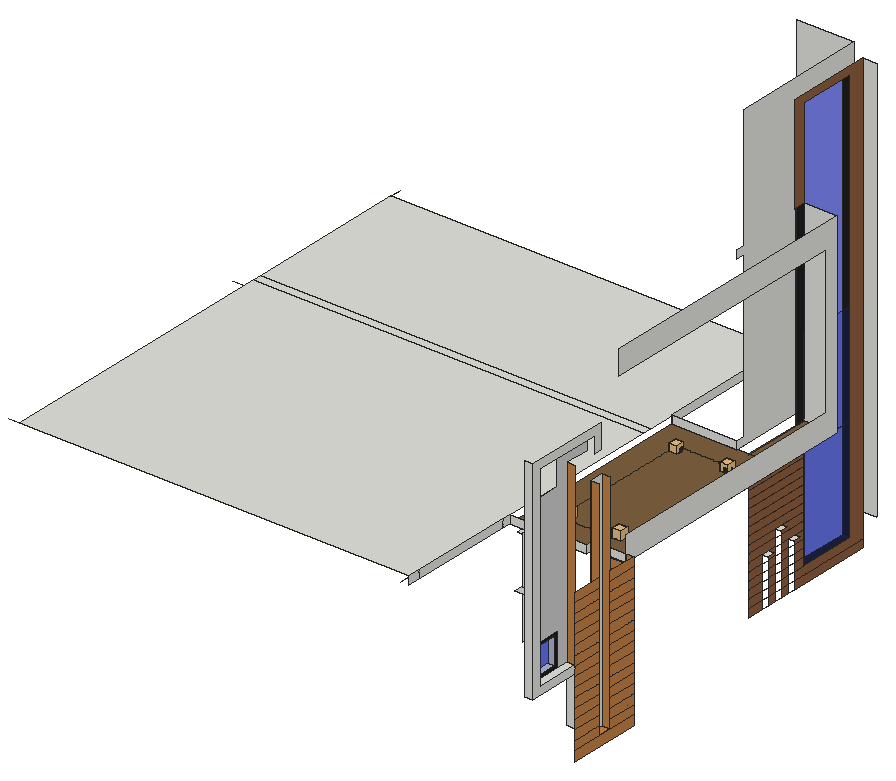
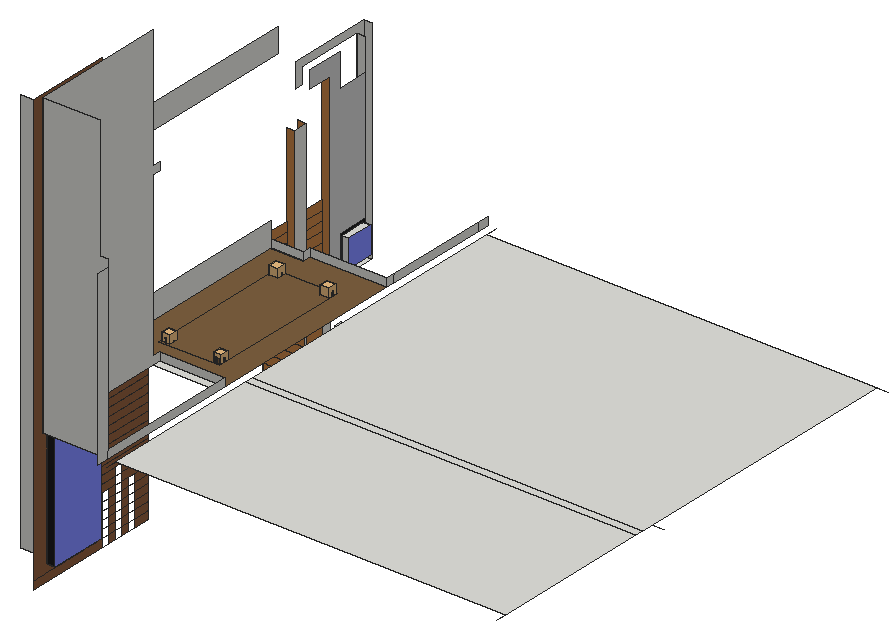
# SketchUp Ruby script. Lengths in inches.
U = 1.inch
M = Sketchup.active_model
def pt(a) = Geom::Point3d.new(a.map { |v| v * U })
def face(e, loops, mat)
  f = e.add_face(loops[0].map { |a| pt(a) })
  loops[1..].each { |l| e.add_face(l.map { |a| pt(a) }).erase! }
  f.material = f.back_material = mat if mat
  f
end
# faces: each face lists its corners as indices into pts; further lists are holes
def faces(e, pts, list, mat = nil) = list.each { |f| face(e, (f[0].is_a?(Array) ? f : [f]).map { |l| l.map { |i| pts[i] } }, mat) }
# xy, xz, yz: faces in a plane at the given z, y or x. An outline is a flat list of corners, or four numbers for a rectangle; further outlines are holes
def ring(l) = l.size == 4 ? [[l[0], l[1]], [l[2], l[1]], [l[2], l[3]], [l[0], l[3]]] : l.each_slice(2).to_a
def flat(e, list, mat, &to3) = list.each { |f| face(e, (f[0].is_a?(Array) ? f : [f]).map { |l| ring(l).map { |u, v| to3.(u, v) } }, mat) }
def xy(e, z, list, mat = nil) = flat(e, list, mat) { |x, y| [x, y, z] }
def xz(e, y, list, mat = nil) = flat(e, list, mat) { |x, z| [x, y, z] }
def yz(e, x, list, mat = nil) = flat(e, list, mat) { |y, z| [x, y, z] }
def lines(e, pts, list) = list.each { |a, b| e.add_line(pt(pts[a]), pt(pts[b])) }
# prism: a flat outline (further loops are holes) pulled along v
def prism(e, loops, v, mat = nil)
  f = face(e, loops, mat); d = Geom::Vector3d.new(v.map { |x| x * U })
  f.pushpull(f.normal.samedirection?(d) ? d.length : -d.length)
end
def box(e, o, s, mat = nil) = prism(e, [[o, [o[0] + s[0], o[1], o[2]], [o[0] + s[0], o[1] + s[1], o[2]], [o[0], o[1] + s[1], o[2]]]], [0, 0, s[2]], mat)
def at(x, y, z, deg = 0) = Geom::Transformation.translation(pt([x, y, z])) * Geom::Transformation.rotation(ORIGIN, Z_AXIS, deg.degrees)
def axes(o, x, y, z) = Geom::Transformation.new([*x, 0, *y, 0, *z, 0, *pt(o).to_a, 1])
def part(name) = M.definitions.add(name)
# library, detail: a bought-in or finely detailed component or shape, given as its bounding box
def library(name, o, s) = part(name).tap { |d| box(d.entities, o, s) }
def detail(e, o, s) = box(e.add_group.entities, o, s)
def put(e, d, t, mat = nil) = e.add_instance(d, t).tap { |i| i.material = mat if mat }
def group(e, t, mat = nil) = e.add_group.tap { |g| g.transformation = t; g.material = mat if mat }.entities
root = M.entities
M.materials.add("E01_Mint_Frost").color = [255, 255, 204]
M.materials.add("Glass_Basic_01").color = [23, 48, 186]
M.materials["Glass_Basic_01"].alpha = 0.25
M.materials.add("I03_Bluebell_Mist").color = [130, 140, 255]
M.materials.add("M08_Obsidian_Black").color = [30, 30, 30]
M.materials.add("Plywood_01_1K").color = [125, 96, 64]
M.materials.add("Wood_Floor_01_1K").color = [196, 130, 70]
M.materials.add("Wood_Veneer_15_1K").color = [142, 95, 62]
M.materials.add("[Cladding_Siding_White]1").color = [207, 207, 207]
c1 = library("Sphere Light\#7",[-3.23,-3.23,-3.23],[6.46,6.46,6.46])
c2 = library("Sphere Light\#4",[-3.22,-3.22,-3.22],[6.44,6.44,6.44])
c3 = library("Sphere Light\#6",[-2.83,-2.83,-2.83],[5.66,5.66,5.66])
c4 = library("Sphere Light\#5",[-2.98,-2.98,-2.98],[5.96,5.96,5.96])
xy(root,171.6,[[384,66.6,390,77.4]],"Wood_Floor_01_1K")
xy(root,174,[[354,294,360,336]],"M08_Obsidian_Black")
xy(root,198,[[360,255,364,261],[360,279,364,285]])
xy(root,210,[[360,267,364,273]])
xy(root,222,[[384,6,390,45]])
xy(root,228,[[384,12,390,45]])
xy(root,230,[[378.546,14,384,34]])
xy(root,231,[[312,87,342,93]],"[Cladding_Siding_White]1")
xy(root,250,[[378.546,14,384,34]])
xy(root,255.544,[[297,108,303,147],[297,151,303,188],[297,192,303,225]])
xy(root,270,[[9,9,297,225],[9,225,297,231],[9,231,297,351],[303,243,351,249]])
xy(root,270,[[[303,93,303,243,384,243,384,99,360,99,360,93],[321,117,366,225]],[[321,117,366,225],[324.799,117.348,325.568,117.497,326.272,117.84,326.864,118.353,327.302,119.002,327.557,119.743,327.613,120.524,327.464,121.293,327.121,121.997,326.607,122.588,325.958,123.027,325.218,123.282,324.437,123.337,323.668,123.188,322.964,122.845,322.372,122.332,321.934,121.683,321.679,120.943,321.624,120.161,321.773,119.393,322.115,118.688,322.629,118.097,323.278,117.659,324.018,117.403],[324.799,217.327,325.568,217.476,326.272,217.819,326.864,218.332,327.302,218.981,327.557,219.722,327.613,220.503,327.464,221.272,327.121,221.976,326.607,222.567,325.958,223.006,325.218,223.261,324.437,223.316,323.668,223.167,322.964,222.824,322.372,222.311,321.934,221.662,321.679,220.922,321.624,220.141,321.773,219.372,322.115,218.668,322.629,218.076,323.278,217.638,324.018,217.382],[362.338,217.327,363.107,217.476,363.811,217.819,364.403,218.332,364.841,218.981,365.097,219.722,365.152,220.503,365.003,221.272,364.66,221.976,364.146,222.567,363.497,223.006,362.757,223.261,361.976,223.316,361.207,223.167,360.503,222.824,359.912,222.311,359.473,221.662,359.218,220.922,359.163,220.141,359.312,219.372,359.654,218.668,360.168,218.076,360.817,217.638,361.557,217.382],[362.338,117.348,363.107,117.497,363.811,117.84,364.403,118.353,364.841,119.002,365.097,119.743,365.152,120.524,365.003,121.293,364.66,121.997,364.146,122.588,363.497,123.027,362.757,123.282,361.976,123.337,361.207,123.188,360.503,122.845,359.912,122.332,359.473,121.683,359.218,120.943,359.163,120.161,359.312,119.393,359.654,118.688,360.168,118.097,360.817,117.659,361.557,117.403]],[360,243,384,294]],"Plywood_01_1K")
xy(root,272.816,[[324.799,217.327,324.018,217.382,323.278,217.638,322.629,218.076,322.115,218.668,321.773,219.372,321.624,220.141,321.679,220.922,321.934,221.662,322.372,222.311,322.964,222.824,323.668,223.167,324.437,223.316,325.218,223.261,325.958,223.006,326.607,222.567,327.121,221.976,327.464,221.272,327.613,220.503,327.557,219.722,327.302,218.981,326.864,218.332,326.272,217.819,325.568,217.476]],"Plywood_01_1K")
xy(root,273,[[324.799,117.348,324.018,117.403,323.278,117.659,322.629,118.097,322.115,118.688,321.773,119.393,321.624,120.161,321.679,120.943,321.934,121.683,322.372,122.332,322.964,122.845,323.668,123.188,324.437,123.337,325.218,123.282,325.958,123.027,326.607,122.588,327.121,121.997,327.464,121.293,327.613,120.524,327.557,119.743,327.302,119.002,326.864,118.353,326.272,117.84,325.568,117.497],[362.338,117.348,361.557,117.403,360.817,117.659,360.168,118.097,359.654,118.688,359.312,119.393,359.163,120.161,359.218,120.943,359.473,121.683,359.912,122.332,360.503,122.845,361.207,123.188,361.976,123.337,362.757,123.282,363.497,123.027,364.146,122.588,364.66,121.997,365.003,121.293,365.152,120.524,365.097,119.743,364.841,119.002,364.403,118.353,363.811,117.84,363.107,117.497],[362.338,217.327,361.557,217.382,360.817,217.638,360.168,218.076,359.654,218.668,359.312,219.372,359.163,220.141,359.218,220.922,359.473,221.662,359.912,222.311,360.503,222.824,361.207,223.167,361.976,223.316,362.757,223.261,363.497,223.006,364.146,222.567,364.66,221.976,365.003,221.272,365.152,220.503,365.097,219.722,364.841,218.981,364.403,218.332,363.811,217.819,363.107,217.476]],"Plywood_01_1K")
xz(root,6,[[384,222,390,378]])
xz(root,12,[[384,228,390,372]])
xz(root,14,[[378.546,230,384,250]])
xz(root,34,[[378.546,230,384,250]])
xz(root,45,[[384,186,390,222]])
xz(root,45,[[384,228,390,360]],"Wood_Floor_01_1K")
xz(root,66.6,[[384,171.6,390,338.4]],"Wood_Floor_01_1K")
xz(root,77.4,[[384,171.6,390,338.4]],"Wood_Floor_01_1K")
xz(root,93,[[303,270,360,276]])
xz(root,99,[[360,270,384,276]])
xz(root,99,[[360,164,384,171],[384,164,390,171],[360,171,384,178],[384,171,390,178],[360,178,384,185],
  [384,178,390,185],[360,185,390,192],[360,192,390,199],[360,199,390,206],[360,206,390,213],
  [360,213,390,220],[360,220,390,227],[360,227,390,234],[360,234,390,241],[360,241,390,248],
  [360,248,390,255],[360,255,390,262],[360,262,390,269],[360,269,360,270,384,270,384,276,390,276,390,269]],"Wood_Floor_01_1K")
xz(root,147,[[297,189.544,303,255.544]])
xz(root,192,[[297,189.544,303,255.544]])
xz(root,243,[[303,270,351,276]])
xz(root,294,[[360,270,384,414]])
xz(root,294,[[354,174,360,480]],"M08_Obsidian_Black")
xz(root,336,[[354,174,360,480]],"M08_Obsidian_Black")
xz(root,348,[[360,186,370,486]])
xz(root,351,[[303,270,351,270,351,492,309,492,309,402,303,402]])
yz(root,303,[[0,270,9,276],[9,270,87,276],[87,270,93,276],[243,270,351,276],[351,270,360,396]])
yz(root,303,[[105,186.544,108,186.544,108,255.544,147,255.544,147,186.544,151,186.544,151,255.544,188,255.544,188,186.544,192,186.544,192,258.544,105,258.544],[192,258.509,231,258.544]],"E01_Mint_Frost")
yz(root,351,[[243,270,243,276,249,276,249,396,243,396,243,402,249,402,249,492,351,492,351,270]])
yz(root,354,[[294,174,336,480]],"I03_Bluebell_Mist")
yz(root,360,[[93,270,99,276]])
yz(root,360,[[294,174,336,250.5],[294,250.5,336,327]],"Glass_Basic_01")
yz(root,360,[[243,162,255,168],[261,162,267,168],[273,162,279,168],[285,162,348,168],[243,168,255,174],
  [285,168,348,168,348,486,285,486,285,414,294,414,294,480,336,480,336,174,294,174,294,270,243,270,243,210,273,210,273,198,285,198],[261,168,267,174],[273,168,279,174],[243,174,255,180],[261,174,267,180],
  [273,174,279,180],[243,180,255,186],[261,180,267,186],[273,180,279,186],[243,186,255,192],
  [261,186,267,192],[273,186,279,192],[243,192,255,198],[261,192,267,198],[273,192,279,198],
  [243,198,267,204],[243,204,267,210]],"Wood_Veneer_15_1K")
yz(root,378.546,[[14,230,34,250]],"I03_Bluebell_Mist")
yz(root,384,[[66.6,171.6,77.4,338.4],[99,270,294,270,294,414,93,414,93,396,283.951,396,283.951,288,99,288]])
yz(root,384,[[14,230,34,250]],"Glass_Basic_01")
yz(root,384,[[[12,228,36,252],[14,230,34,250]]],"M08_Obsidian_Black")
yz(root,384,[[36,228,45,228,45,360,63,360,63,372,36,372,36,348,12,348,12,252,36,252]],"[Cladding_Siding_White]1")
yz(root,390,[[6,222,45,222,45,228,12,228,12,372,63,372,63,360,69,360,69,378,6,378]])
yz(root,390,[[45,164,99,171],[45,171,99,171,99,178,77.4,178,77.4,171.6,66.6,171.6,66.6,178,45,178],[45,178,66.6,185],[77.4,178,99,185],[45,185,66.6,192],
  [77.4,185,99,192],[45,192,66.6,199],[77.4,192,99,199],[45,199,66.6,206],[77.4,199,99,206],
  [45,206,66.6,213],[77.4,206,99,213],[45,213,66.6,220],[77.4,213,99,220],[45,220,66.6,227],
  [77.4,220,99,227],[45,227,66.6,234],[77.4,227,99,234],[45,234,66.6,241],[77.4,234,99,241],
  [45,241,66.6,248],[77.4,241,99,248],[45,248,66.6,255],[77.4,248,99,255],[45,255,66.6,262],
  [77.4,255,99,262],[45,262,66.6,269],[77.4,262,99,269],[45,269,66.6,276],[77.4,269,99,276]],"Wood_Floor_01_1K")
p = [[324.799,117.348,270],[324.018,117.403,270],[324.018,117.403,273],[324.799,117.348,273],[325.568,117.497,270],[325.568,117.497,273],
  [362.338,117.348,270],[361.557,117.403,270],[361.557,117.403,273],[362.338,117.348,273],[363.107,117.497,270],[363.107,117.497,273],
  [323.278,117.659,270],[323.278,117.659,273],[360.817,117.659,270],[360.817,117.659,273],[326.272,117.84,270],[326.272,117.84,273],
  [363.811,117.84,270],[363.811,117.84,273],[322.629,118.097,270],[322.629,118.097,273],[360.168,118.097,270],[360.168,118.097,273],
  [326.864,118.353,270],[326.864,118.353,273],[364.403,118.353,270],[364.403,118.353,273],[322.115,118.688,270],[322.115,118.688,273],
  [359.654,118.688,270],[359.654,118.688,273],[327.302,119.002,270],[327.302,119.002,273],[364.841,119.002,270],[364.841,119.002,273],
  [321.773,119.393,270],[321.773,119.393,273],[359.312,119.393,270],[359.312,119.393,273],[327.557,119.743,270],[327.557,119.743,273],
  [365.097,119.743,270],[365.097,119.743,273],[321.624,120.161,270],[321.624,120.161,273],[359.163,120.161,270],[359.163,120.161,273],
  [327.613,120.524,270],[327.613,120.524,273],[365.152,120.524,270],[365.152,120.524,273],[321.679,120.943,270],[321.679,120.943,273],
  [359.218,120.943,270],[359.218,120.943,273],[327.464,121.293,270],[327.464,121.293,273],[365.003,121.293,270],[365.003,121.293,273],
  [321.934,121.683,270],[321.934,121.683,273],[359.473,121.683,270],[359.473,121.683,273],[327.121,121.997,270],[327.121,121.997,273],
  [364.66,121.997,270],[364.66,121.997,273],[322.372,122.332,270],[322.372,122.332,273],[359.912,122.332,270],[359.912,122.332,273],
  [326.607,122.588,270],[326.607,122.588,273],[364.146,122.588,270],[364.146,122.588,273],[322.964,122.845,270],[322.964,122.845,273],
  [360.503,122.845,270],[360.503,122.845,273],[325.958,123.027,270],[325.958,123.027,273],[363.497,123.027,270],[363.497,123.027,273],
  [323.668,123.188,270],[323.668,123.188,273],[361.207,123.188,270],[361.207,123.188,273],[325.218,123.282,270],[325.218,123.282,273],
  [362.757,123.282,270],[362.757,123.282,273],[324.437,123.337,270],[324.437,123.337,273],[361.976,123.337,270],[361.976,123.337,273],
  [324.799,217.327,270],[324.018,217.382,270],[324.018,217.382,272.816],[324.799,217.327,272.816],[325.568,217.476,270],[325.568,217.476,272.816],
  [362.338,217.327,270],[361.557,217.382,270],[361.557,217.382,273],[362.338,217.327,273],[363.107,217.476,270],[363.107,217.476,273],
  [323.278,217.638,270],[323.278,217.638,272.816],[360.817,217.638,270],[360.817,217.638,273],[326.272,217.819,270],[326.272,217.819,272.816],
  [363.811,217.819,270],[363.811,217.819,273],[322.629,218.076,270],[322.629,218.076,272.816],[360.168,218.076,270],[360.168,218.076,273],
  [326.864,218.332,270],[326.864,218.332,272.816],[364.403,218.332,270],[364.403,218.332,273],[322.115,218.668,270],[322.115,218.668,272.816],
  [359.654,218.668,270],[359.654,218.668,273],[327.302,218.981,270],[327.302,218.981,272.816],[364.841,218.981,270],[364.841,218.981,273],
  [321.773,219.372,270],[321.773,219.372,272.816],[359.312,219.372,270],[359.312,219.372,273],[327.557,219.722,270],[327.557,219.722,272.816],
  [365.097,219.722,270],[365.097,219.722,273],[321.624,220.141,270],[321.624,220.141,272.816],[359.163,220.141,270],[359.163,220.141,273],
  [327.613,220.503,270],[327.613,220.503,272.816],[365.152,220.503,270],[365.152,220.503,273],[321.679,220.922,270],[321.679,220.922,272.816],
  [359.218,220.922,270],[359.218,220.922,273],[327.464,221.272,270],[327.464,221.272,272.816],[365.003,221.272,270],[365.003,221.272,273],
  [321.934,221.662,270],[321.934,221.662,272.816],[359.473,221.662,270],[359.473,221.662,273],[327.121,221.976,270],[327.121,221.976,272.816],
  [364.66,221.976,270],[364.66,221.976,273],[322.372,222.311,270],[322.372,222.311,272.816],[359.912,222.311,270],[359.912,222.311,273],
  [326.607,222.567,270],[326.607,222.567,272.816],[364.146,222.567,270],[364.146,222.567,273],[322.964,222.824,270],[322.964,222.824,272.816],
  [360.503,222.824,270],[360.503,222.824,273],[325.958,223.006,270],[325.958,223.006,272.816],[363.497,223.006,270],[363.497,223.006,273],
  [323.668,223.167,270],[323.668,223.167,272.816],[361.207,223.167,270],[361.207,223.167,273],[325.218,223.261,270],[325.218,223.261,272.816],
  [362.757,223.261,270],[362.757,223.261,273],[324.437,223.316,270],[324.437,223.316,272.816],[361.976,223.316,270],[361.976,223.316,273],
  [297,9,270],[297,0,270],[9,216,270],[0,216,270],[9,9,270],[0,9,270],
  [9,351,270],[9,360,270],[297,351,270],[297,360,270],[384,93,180],[390,93,180],
  [303.145,190.706,258.509],[303,231,258.509],[303,192,258.509],[303,190.706,258.509],[360,242.998,264],[360,243,264],
  [360,293.998,264],[360,242.996,258],[360,243,258],[360,293.996,258],[360,242.994,252],[360,243,252],
  [360,293.994,252],[360,242.992,246],[360,243,246],[360,293.992,246],[360,242.99,240],[360,243,240],
  [360,293.99,240],[360,242.988,234],[360,243,234],[360,293.988,234],[360,242.986,228],[360,243,228],
  [360,293.986,228],[360,242.984,222],[360,243,222],[360,293.984,222],[360,242.982,216],[360,243,216],
  [360,293.982,216],[360,242.98,210],[360,243,210],[360,273,210],[360,293.98,210],[360,242.978,204],
  [360,243,204],[360,267,204],[360,273,204],[360,293.978,204],[360,242.976,198],[360,243,198],
  [360,285,198],[360,293.976,198],[360,267,198],[360,273,198],[360,242.975,192],[360,243,192],
  [360,255,192],[360,261,192],[360,267,192],[360,273,192],[360,279,192],[360,285,192],
  [360,293.975,192],[360,242.973,186],[360,243,186],[360,255,186],[360,261,186],[360,267,186],
  [360,273,186],[360,279,186],[360,285,186],[360,293.973,186],[360,242.971,180],[360,243,180],
  [360,255,180],[360,261,180],[360,267,180],[360,273,180],[360,279,180],[360,285,180],
  [360,293.971,180],[360,242.969,174],[360,243,174],[360,255,174],[360,261,174],[360,267,174],
  [360,273,174],[360,279,174],[360,285,174],[360,293.969,174],[360,242.967,168],[360,243,168],
  [360,255,168],[360,261,168],[360,267,168],[360,273,168],[360,279,168],[360,285,168],
  [360,242.965,162],[360,243,162],[360,255,162],[360,261,162],[360,267,162],[360,273,162],
  [360,279,162],[360,285,162]]
faces(root,p,[[0,1,2,3],[4,0,3,5],[6,7,8,9],[10,6,9,11],[1,12,13,2],[7,14,15,8],[16,4,5,17],[18,10,11,19],
  [12,20,21,13],[14,22,23,15],[24,16,17,25],[26,18,19,27],[20,28,29,21],[22,30,31,23],[32,24,25,33],[34,26,27,35],
  [28,36,37,29],[30,38,39,31],[40,32,33,41],[42,34,35,43],[36,44,45,37],[38,46,47,39],[48,40,41,49],[50,42,43,51],
  [44,52,53,45],[46,54,55,47],[56,48,49,57],[58,50,51,59],[52,60,61,53],[54,62,63,55],[64,56,57,65],[66,58,59,67],
  [60,68,69,61],[62,70,71,63],[72,64,65,73],[74,66,67,75],[68,76,77,69],[70,78,79,71],[80,72,73,81],[82,74,75,83],
  [76,84,85,77],[78,86,87,79],[88,80,81,89],[90,82,83,91],[84,92,93,85],[86,94,95,87],[92,88,89,93],[94,90,91,95],
  [96,97,98,99],[100,96,99,101],[102,103,104,105],[106,102,105,107],[97,108,109,98],[103,110,111,104],[112,100,101,113],[114,106,107,115],
  [108,116,117,109],[110,118,119,111],[120,112,113,121],[122,114,115,123],[116,124,125,117],[118,126,127,119],[128,120,121,129],[130,122,123,131],
  [124,132,133,125],[126,134,135,127],[136,128,129,137],[138,130,131,139],[132,140,141,133],[134,142,143,135],[144,136,137,145],[146,138,139,147],
  [140,148,149,141],[142,150,151,143],[152,144,145,153],[154,146,147,155],[148,156,157,149],[150,158,159,151],[160,152,153,161],[162,154,155,163],
  [156,164,165,157],[158,166,167,159],[168,160,161,169],[170,162,163,171],[164,172,173,165],[166,174,175,167],[176,168,169,177],[178,170,171,179],
  [172,180,181,173],[174,182,183,175],[184,176,177,185],[186,178,179,187],[180,188,189,181],[182,190,191,183],[188,184,185,189],[190,186,187,191]],"Plywood_01_1K")
lines(root,p,[[192,193],[194,195],[196,197],[198,199],[200,201],[202,203],[204,205],[206,207],[208,209],[209,210],[211,212],[212,213],
  [214,215],[215,216],[217,218],[218,219],[220,221],[221,222],[223,224],[224,225],[226,227],[227,228],[229,230],[230,231],
  [232,233],[233,234],[235,236],[237,238],[239,240],[241,242],[242,243],[244,245],[246,247],[248,249],[250,251],[252,253],
  [254,255],[256,257],[257,258],[259,260],[261,262],[263,264],[265,266],[266,267],[268,269],[270,271],[272,273],[274,275],
  [275,276],[277,278],[279,280],[281,282],[283,284],[284,285],[286,287],[288,289],[290,291],[292,293],[294,295],[296,297],
  [298,299],[300,301]])
put(root,c1,at(324.96,120.3125,273))
put(root,c2,at(362.39,120.4,273))
put(root,c3,at(324.57,220.02,272.82))
put(root,c4,at(362.1,220.41,273))
